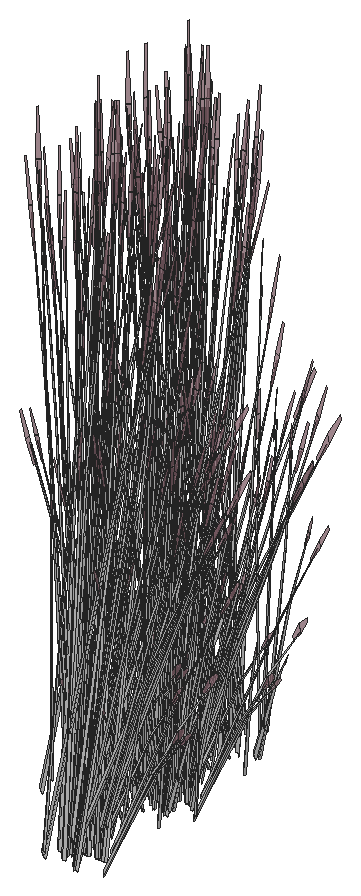
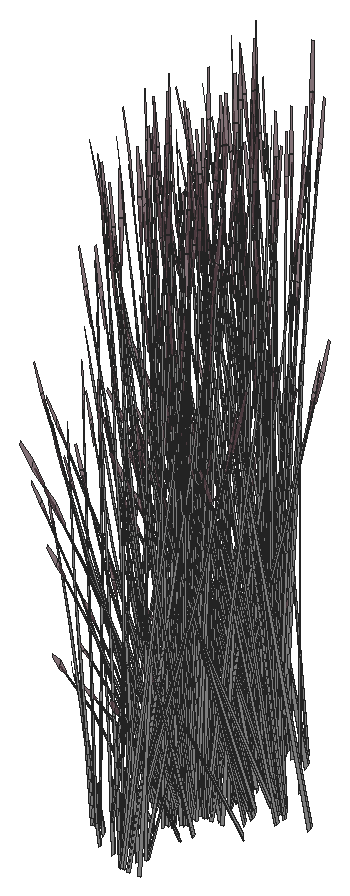
# SketchUp Ruby script. Lengths in inches.
U = 1.inch
M = Sketchup.active_model
def pt(a) = Geom::Point3d.new(a.map { |v| v * U })
def face(e, loops, mat)
  f = e.add_face(loops[0].map { |a| pt(a) })
  loops[1..].each { |l| e.add_face(l.map { |a| pt(a) }).erase! }
  f.material = f.back_material = mat if mat
  f
end
# faces: each face lists its corners as indices into pts; further lists are holes
def faces(e, pts, list, mat = nil) = list.each { |f| face(e, (f[0].is_a?(Array) ? f : [f]).map { |l| l.map { |i| pts[i] } }, mat) }
# xy, xz, yz: faces in a plane at the given z, y or x. An outline is a flat list of corners, or four numbers for a rectangle; further outlines are holes
def ring(l) = l.size == 4 ? [[l[0], l[1]], [l[2], l[1]], [l[2], l[3]], [l[0], l[3]]] : l.each_slice(2).to_a
def flat(e, list, mat, &to3) = list.each { |f| face(e, (f[0].is_a?(Array) ? f : [f]).map { |l| ring(l).map { |u, v| to3.(u, v) } }, mat) }
def xy(e, z, list, mat = nil) = flat(e, list, mat) { |x, y| [x, y, z] }
def xz(e, y, list, mat = nil) = flat(e, list, mat) { |x, z| [x, y, z] }
def yz(e, x, list, mat = nil) = flat(e, list, mat) { |y, z| [x, y, z] }
def lines(e, pts, list) = list.each { |a, b| e.add_line(pt(pts[a]), pt(pts[b])) }
# prism: a flat outline (further loops are holes) pulled along v
def prism(e, loops, v, mat = nil)
  f = face(e, loops, mat); d = Geom::Vector3d.new(v.map { |x| x * U })
  f.pushpull(f.normal.samedirection?(d) ? d.length : -d.length)
end
def box(e, o, s, mat = nil) = prism(e, [[o, [o[0] + s[0], o[1], o[2]], [o[0] + s[0], o[1] + s[1], o[2]], [o[0], o[1] + s[1], o[2]]]], [0, 0, s[2]], mat)
def at(x, y, z, deg = 0) = Geom::Transformation.translation(pt([x, y, z])) * Geom::Transformation.rotation(ORIGIN, Z_AXIS, deg.degrees)
def axes(o, x, y, z) = Geom::Transformation.new([*x, 0, *y, 0, *z, 0, *pt(o).to_a, 1])
def part(name) = M.definitions.add(name)
# library, detail: a bought-in or finely detailed component or shape, given as its bounding box
def library(name, o, s) = part(name).tap { |d| box(d.entities, o, s) }
def detail(e, o, s) = box(e.add_group.entities, o, s)
def put(e, d, t, mat = nil) = e.add_instance(d, t).tap { |i| i.material = mat if mat }
def group(e, t, mat = nil) = e.add_group.tap { |g| g.transformation = t; g.material = mat if mat }.entities
root = M.entities
M.materials.add("LightPink_Translucent").color = [144, 107, 117]
M.materials["LightPink_Translucent"].alpha = 0.75
M.materials.add("[_0053_Ivory_]").color = [200, 200, 200]
c1 = part("blade")
p = [[2.15,0.21,22],[0,0.17,0],[0.09,0.45,0],[2.18,0.31,22],[2.29,0.31,22],[0.38,0.45,0],
  [2.48,0.24,33],[2.49,0.24,33],[2.48,0.22,33]]
faces(c1.entities,p,[[0,1,2,3],[4,5,2,3],[6,3,4,7],[8,0,3,6]])
c2 = part("seeds")
p = [[0.3,-0.1,1.38],[-0.01,-0.03,1.59],[-0.01,-0.03,0.03],[0.14,-0.07,-0.07],[0.29,-0.03,3],[0.15,0.01,3.11]]
faces(c2.entities,p,[[0,1,2,3],[1,0,4,5]],"LightPink_Translucent")
c3 = part("blade with seeds")
put(c3.entities,c1,at(0,0,0))
put(c3.entities,c2,axes([2.4,0.25,30.99],[1.5799,-0.05474,1.17369],[-0.12525,1.92788,0.29478],[-0.07173,-0.02425,1.56792]))
put(root,c3,axes([678.38,324.65,38.66],[0.43478,0.42253,-0.5672],[-0.45929,0.37004,-0.43934],[-0.06615,0.21468,1.08528]),"[_0053_Ivory_]")
put(root,c3,axes([680.62,314.26,35.68],[-0.56663,-0.1556,-0.30978],[0.14267,-0.54795,0.30978],[-0.11423,0.06319,1.38974]),"[_0053_Ivory_]")
put(root,c3,axes([680.62,324.85,35.68],[-0.56663,-0.1556,-0.30978],[0.14267,-0.54795,0.30978],[-0.11423,0.06319,1.38974]),"[_0053_Ivory_]")
put(root,c3,axes([674.08,318.79,36.32],[0.61322,-0.4175,-0.29095],[0.40778,0.58992,-0.50002],[0.1513,0.05991,1.59708]),"[_0053_Ivory_]")
put(root,c3,axes([675.55,322.3,36.32],[-0.38947,-0.01972,1.0506],[0.25721,-0.41888,0.58006],[0.15386,0.14882,0.8241]),"[_0053_Ivory_]")
put(root,c3,axes([679.16,322.7,36.32],[-0.68399,-0.30005,-0.29095],[0.32934,-0.63331,-0.50002],[-0.0215,-0.15549,1.59708]),"[_0053_Ivory_]")
put(root,c3,axes([679.16,332.84,36.32],[-0.68399,-0.30005,-0.29095],[0.32934,-0.63331,-0.50002],[-0.0215,-0.15549,1.59708]),"[_0053_Ivory_]")
put(root,c3,axes([680.94,311.92,36.5],[-0.01659,-0.59209,1.41272],[0.75089,0.15348,0.59816],[-0.1776,0.32398,1.3335]),"[_0053_Ivory_]")
put(root,c3,axes([680.94,322.51,36.5],[-0.01659,-0.59209,1.41272],[0.75089,0.15348,0.59816],[-0.1776,0.32398,1.3335]),"[_0053_Ivory_]")
put(root,c3,axes([674.38,317.28,37.53],[-0.11309,0.21615,1.71376],[-0.47441,-0.44731,0.13857],[0.21402,-0.27879,0.73262]),"[_0053_Ivory_]")
put(root,c3,axes([677.91,314.6875,36.48],[0.55175,-0.11136,0.06507],[0.12684,0.44864,-0.86304],[-0.03498,0.22711,0.7736]),"[_0053_Ivory_]")
put(root,c3,axes([677.91,325.28,36.48],[0.55175,-0.11136,0.06507],[0.12684,0.44864,-0.86304],[-0.03498,0.22711,0.7736]),"[_0053_Ivory_]")
put(root,c3,axes([680.52,312.67,36.32],[0.07077,0.71755,-0.29095],[-0.73712,0.04339,-0.50002],[-0.1298,0.09558,1.59708]),"[_0053_Ivory_]")
put(root,c3,axes([680.52,323.26,36.32],[0.07077,0.71755,-0.29095],[-0.73712,0.04339,-0.50002],[-0.1298,0.09558,1.59708]),"[_0053_Ivory_]")
put(root,c3,axes([678.86,322.06,35.75],[-0.24943,-0.64486,-0.69835],[0.71849,-0.23224,-0.18329],[-0.02757,-0.21836,1.54149]),"[_0053_Ivory_]")
put(root,c3,axes([678.86,332.2,35.75],[-0.24943,-0.64486,-0.69835],[0.71849,-0.23224,-0.18329],[-0.02757,-0.21836,1.54149]),"[_0053_Ivory_]")
put(root,c3,axes([679.98,320.04,38.33],[-0.59704,-0.15764,-0.51099],[0.20464,-0.54049,-0.3958],[-0.05475,-0.21761,0.97773]),"[_0053_Ivory_]")
put(root,c3,axes([679.98,330.18,38.33],[-0.59704,-0.15764,-0.51099],[0.20464,-0.54049,-0.3958],[-0.05475,-0.21761,0.97773]),"[_0053_Ivory_]")
put(root,c3,axes([678.88,313.45,37.53],[-0.01487,-0.24136,1.71376],[0.64429,0.16012,0.13857],[-0.03985,0.34396,0.73262]),"[_0053_Ivory_]")
put(root,c3,axes([672.53,318.41,35.25],[-0.59782,0.25177,1.28929],[-0.19028,-0.72239,0.50096],[0.36709,0.01202,1.46642]),"[_0053_Ivory_]")
put(root,c3,axes([677.68,321.98,35.68],[0.42396,-0.39235,-0.30978],[0.42396,0.39235,0.30978],[0,-0.12637,1.38974]),"[_0053_Ivory_]")
put(root,c3,axes([677.68,332.12,35.68],[0.42396,-0.39235,-0.30978],[0.42396,0.39235,0.30978],[0,-0.12637,1.38974]),"[_0053_Ivory_]")
put(root,c3,axes([679.59,319.45,35.78],[-0.4197,0.36076,-0.03893],[-0.38456,-0.39511,-0.17649],[-0.02707,-0.11196,0.58215]),"[_0053_Ivory_]")
put(root,c3,axes([679.59,329.59,35.78],[-0.4197,0.36076,-0.03893],[-0.38456,-0.39511,-0.17649],[-0.02707,-0.11196,0.58215]),"[_0053_Ivory_]")
put(root,c3,axes([679.42,312.41,36.01],[0.76764,0.13249,0.45755],[-0.15622,0.74829,0.17955],[-0.11218,-0.07226,1.58856]),"[_0053_Ivory_]")
put(root,c3,axes([679.42,323,36.01],[0.76764,0.13249,0.45755],[-0.15622,0.74829,0.17955],[-0.11218,-0.07226,1.58856]),"[_0053_Ivory_]")
put(root,c3,axes([674.73,321.73,38.33],[0.59932,-0.14948,-0.51099],[0.10484,0.56611,-0.3958],[0.16097,0.16223,0.97773]),"[_0053_Ivory_]")
put(root,c3,axes([675.28,317.3,36.03],[0.37973,-0.63014,0],[0.6353,0.35142,-0.51607],[0.14469,0.08004,1.63711]),"[_0053_Ivory_]")
put(root,c3,axes([675.91,317.02,35.15],[-0.0909,-0.04954,1.76342],[-0.2335,-0.55347,-0.26939],[0.15752,-0.1502,0.30037]),"[_0053_Ivory_]")
put(root,c3,axes([679.22,322.87,36.37],[-0.29468,0.56664,0.44739],[-0.61229,-0.27271,-0.21531],[0,-0.13062,1.43643]),"[_0053_Ivory_]")
put(root,c3,axes([680.2,320.14,38.63],[-0.28988,-0.51132,-0.71045],[0.59671,-0.28496,0.08574],[-0.06778,-0.24706,1.00501]),"[_0053_Ivory_]")
put(root,c3,axes([680.2,330.28,38.63],[-0.28988,-0.51132,-0.71045],[0.59671,-0.28496,0.08574],[-0.06778,-0.24706,1.00501]),"[_0053_Ivory_]")
put(root,c3,axes([675.625,317.68,35.67],[0.56842,0.31443,-0.49651],[-0.33976,0.56381,0],[0.12946,0.07161,1.57504]),"[_0053_Ivory_]")
put(root,c3,axes([675.6,322.15,35.15],[0.04425,-0.09079,1.76342],[0.55709,-0.26738,-0.26939],[0.16889,0.13839,0.30037]),"[_0053_Ivory_]")
put(root,c3,axes([675.9,318.35,38.33],[-0.15602,-0.5742,-0.51099],[0.59087,-0.10045,-0.3958],[0.16933,-0.15423,0.97773]),"[_0053_Ivory_]")
put(root,c3,axes([679.01,313.61,36.13],[0.65264,-0.16691,0.17642],[0.16115,0.62115,0.35086],[-0.05821,-0.0905,1.60407]),"[_0053_Ivory_]")
put(root,c3,axes([679.01,324.2,36.13],[0.65264,-0.16691,0.17642],[0.16115,0.62115,0.35086],[-0.05821,-0.0905,1.60407]),"[_0053_Ivory_]")
put(root,c3,axes([676.93,321.3125,37.58],[-0.11624,-0.52862,-0.03492],[0.54943,-0.12153,-0.15832],[0.11473,0.03351,0.52218]),"[_0053_Ivory_]")
put(root,c3,axes([679.85,313.71,35.85],[-0.61229,-0.28233,0],[0.29468,-0.58663,0],[0,0,1.62707]),"[_0053_Ivory_]")
put(root,c3,axes([679.85,324.3,35.85],[-0.61229,-0.28233,0],[0.29468,-0.58663,0],[0,0,1.62707]),"[_0053_Ivory_]")
put(root,c3,axes([681.27,314.41,36.03],[0.37973,0.63014,0],[-0.6353,0.35142,-0.51607],[-0.14469,0.08004,1.63711]),"[_0053_Ivory_]")
put(root,c3,axes([681.27,325,36.03],[0.37973,0.63014,0],[-0.6353,0.35142,-0.51607],[-0.14469,0.08004,1.63711]),"[_0053_Ivory_]")
put(root,c3,axes([674.8,318.88,35.71],[0.63179,0.1031,-0.62353],[-0.13332,0.63596,-0.16365],[0.18854,0.07706,1.37633]),"[_0053_Ivory_]")
put(root,c3,axes([677.49,319.25,35.91],[-0.37654,-0.40212,-0.06488],[0.4124,-0.36845,-0.29416],[0.11685,-0.02594,0.97024]),"[_0053_Ivory_]")
put(root,c3,axes([676.62,317.21,36.42],[-0.2023,0.32011,1.1486],[-0.17388,-0.43009,0.84392],[0.16708,-0.10777,0.25299]),"[_0053_Ivory_]")
put(root,c3,axes([680.95,313.64,36.13],[0.17545,-0.62497,0.17642],[0.64204,0.17686,0.35086],[-0.11091,0.00304,1.60407]),"[_0053_Ivory_]")
put(root,c3,axes([680.95,324.23,36.13],[0.17545,-0.62497,0.17642],[0.64204,0.17686,0.35086],[-0.11091,0.00304,1.60407]),"[_0053_Ivory_]")
put(root,c3,axes([680.66,312.8125,36.27],[0.44871,0.37783,0.1448],[-0.37428,0.42627,-0.41347],[-0.10418,0.05763,1.26744]),"[_0053_Ivory_]")
put(root,c3,axes([680.66,323.4,36.27],[0.44871,0.37783,0.1448],[-0.37428,0.42627,-0.41347],[-0.10418,0.05763,1.26744]),"[_0053_Ivory_]")
put(root,c3,axes([680.5,312.34,35.95],[-0.56493,-0.54126,-0.06131],[0.56528,-0.54159,0],[-0.01973,-0.0189,1.75571]),"[_0053_Ivory_]")
put(root,c3,axes([680.5,322.9375,35.95],[-0.56493,-0.54126,-0.06131],[0.56528,-0.54159,0],[-0.01973,-0.0189,1.75571]),"[_0053_Ivory_]")
put(root,c3,axes([680.65,312.53,36.37],[0.65953,-0.03882,0.44739],[0.05964,0.64439,-0.21531],[-0.11807,0.06531,1.43643]),"[_0053_Ivory_]")
put(root,c3,axes([680.65,323.125,36.37],[0.65953,-0.03882,0.44739],[0.05964,0.64439,-0.21531],[-0.11807,0.06531,1.43643]),"[_0053_Ivory_]")
put(root,c3,axes([680.81,314.02,35.98],[0.76036,0.2044,0.30756],[-0.19023,0.7306,-0.36492],[-0.12585,0.09144,1.64885]),"[_0053_Ivory_]")
put(root,c3,axes([680.81,324.61,35.98],[0.76036,0.2044,0.30756],[-0.19023,0.7306,-0.36492],[-0.12585,0.09144,1.64885]),"[_0053_Ivory_]")
put(root,c3,axes([679.7,319,35.15],[-0.10187,0.02266,1.76342],[-0.56336,-0.25503,-0.26939],[0.00945,-0.21273,0.30037]),"[_0053_Ivory_]")
put(root,c3,axes([679.7,329.14,35.15],[-0.10187,0.02266,1.76342],[-0.56336,-0.25503,-0.26939],[0.00945,-0.21273,0.30037]),"[_0053_Ivory_]")
put(root,c3,axes([681.13,313.98,36.13],[0.56842,-0.31443,0.49651],[0.33976,0.56381,0],[-0.12946,0.07161,1.57504]),"[_0053_Ivory_]")
put(root,c3,axes([681.13,324.57,36.13],[0.56842,-0.31443,0.49651],[0.33976,0.56381,0],[-0.12946,0.07161,1.57504]),"[_0053_Ivory_]")
put(root,c3,axes([674.66,320.24,37.53],[-0.2256,-0.10835,1.71376],[0.46687,-0.45453,0.13857],[0.29098,0.20505,0.73262]),"[_0053_Ivory_]")
put(root,c3,axes([680.25,319.7,38.18],[0.1831,-0.48359,-0.35414],[0.53419,0.14105,0.4572],[-0.04898,-0.1947,0.87481]),"[_0053_Ivory_]")
put(root,c3,axes([680.25,329.84,38.18],[0.1831,-0.48359,-0.35414],[0.53419,0.14105,0.4572],[-0.04898,-0.1947,0.87481]),"[_0053_Ivory_]")
put(root,c3,axes([679.36,322.31,36.01],[0.26406,0.70318,0.45755],[-0.7545,0.24452,0.17955],[0.00922,-0.12921,1.58856]),"[_0053_Ivory_]")
put(root,c3,axes([679.24,322.23,35.86],[0.29468,-0.56664,-0.44739],[0.61229,0.27271,0.21531],[0,-0.13062,1.43643]),"[_0053_Ivory_]")
put(root,c3,axes([679.24,332.37,35.86],[0.29468,-0.56664,-0.44739],[0.61229,0.27271,0.21531],[0,-0.13062,1.43643]),"[_0053_Ivory_]")
put(root,c3,axes([679.99,313.46,35.86],[-0.19817,-0.54216,0],[0.56587,-0.18986,0],[0,0,1.54371]),"[_0053_Ivory_]")
put(root,c3,axes([679.99,324.05,35.86],[-0.19817,-0.54216,0],[0.56587,-0.18986,0],[0,0,1.54371]),"[_0053_Ivory_]")
put(root,c3,axes([679.27,314.6,35.15],[0.09829,-0.03422,1.76342],[0.59126,0.18834,-0.26939],[0.01729,0.21228,0.30037]),"[_0053_Ivory_]")
put(root,c3,axes([679.27,325.2,35.15],[0.09829,-0.03422,1.76342],[0.59126,0.18834,-0.26939],[0.01729,0.21228,0.30037]),"[_0053_Ivory_]")
put(root,c3,axes([676.33,318.41,38.18],[0.52868,-0.08987,-0.35414],[0.1396,0.51376,0.4572],[0.1515,-0.13799,0.87481]),"[_0053_Ivory_]")
put(root,c3,axes([679.4,314.8,38.18],[-0.1831,0.48359,-0.35414],[-0.53419,-0.14105,0.4572],[0.04898,0.1947,0.87481]),"[_0053_Ivory_]")
put(root,c3,axes([675.91,318.58,38.63],[0.31725,-0.49618,-0.71045],[0.55593,0.35263,0.08574],[0.18942,-0.17977,1.00501]),"[_0053_Ivory_]")
put(root,c3,axes([675.91,321.25,38.18],[0.34557,0.39372,-0.35414],[-0.39459,0.37271,0.4572],[0.20048,0.05671,0.87481]),"[_0053_Ivory_]")
put(root,c3,axes([680.79,312.39,35.86],[-0.29468,0.56664,-0.44739],[-0.61229,-0.27271,0.21531],[0,0.13062,1.43643]),"[_0053_Ivory_]")
put(root,c3,axes([680.79,322.98,35.86],[-0.29468,0.56664,-0.44739],[-0.61229,-0.27271,0.21531],[0,0.13062,1.43643]),"[_0053_Ivory_]")
put(root,c3,axes([681.95,312.05,36.13],[-0.47719,-0.45806,0.17642],[0.48088,-0.44429,0.35086],[-0.0527,0.09355,1.60407]),"[_0053_Ivory_]")
put(root,c3,axes([681.95,322.64,36.13],[-0.47719,-0.45806,0.17642],[0.48088,-0.44429,0.35086],[-0.0527,0.09355,1.60407]),"[_0053_Ivory_]")
put(root,c3,axes([680.31,322.375,35.86],[0,-0.72763,0],[0.75945,0,0],[0,0,1.79456]),"[_0053_Ivory_]")
put(root,c3,axes([679.6,322.51,36.09],[0.68433,0.30479,0.24065],[-0.32934,0.63331,0.50002],[0,-0.14599,1.60543]),"[_0053_Ivory_]")
put(root,c3,axes([680.6875,312.07,35.95],[0,0.72727,-0.05637],[-0.75945,0,0],[0,0.02286,1.79368]),"[_0053_Ivory_]")
put(root,c3,axes([680.6875,322.66,35.95],[0,0.72727,-0.05637],[-0.75945,0,0],[0,0.02286,1.79368]),"[_0053_Ivory_]")
put(root,c3,axes([679.38,322.08,36.37],[-0.65953,0.03882,0.44739],[-0.05964,-0.64439,-0.21531],[0.11807,-0.06531,1.43643]),"[_0053_Ivory_]")
put(root,c3,axes([676.17,319.625,38.33],[0.16454,-0.57202,-0.51099],[0.56413,0.19607,-0.3958],[0.22713,-0.05245,0.97773]),"[_0053_Ivory_]")
put(root,c3,axes([677.59,319.99,36.42],[-0.37526,0.10382,1.1486],[0.17664,-0.42906,0.84392],[0.19907,0.02936,0.25299]),"[_0053_Ivory_]")
put(root,c3,axes([679.07,310.38,36.13],[-0.17545,0.62497,0.17642],[-0.64204,-0.17686,0.35086],[0.11091,-0.00304,1.60407]),"[_0053_Ivory_]")
put(root,c3,axes([679.07,320.98,36.13],[-0.17545,0.62497,0.17642],[-0.64204,-0.17686,0.35086],[0.11091,-0.00304,1.60407]),"[_0053_Ivory_]")
put(root,c3,axes([680.32,313.48,35.94],[0.26406,0.72244,-0.06012],[-0.7545,0.25315,0],[0.00922,0.02523,1.72173]),"[_0053_Ivory_]")
put(root,c3,axes([680.32,324.07,35.94],[0.26406,0.72244,-0.06012],[-0.7545,0.25315,0],[0.00922,0.02523,1.72173]),"[_0053_Ivory_]")
put(root,c3,axes([676.37,318.125,36.24],[-0.21697,-0.01863,1.43002],[-0.22228,-0.49966,-0.30754],[0.26655,-0.14135,0.61141]),"[_0053_Ivory_]")
put(root,c3,axes([676.52,319.89,38.18],[0.50475,0.17543,-0.35414],[-0.14722,0.5118,0.4572],[0.20322,-0.04693,0.87481]),"[_0053_Ivory_]")
put(root,c3,axes([678.76,320.2,36.03],[-0.37973,-0.63014,0],[0.6353,-0.35142,-0.51607],[0.14469,-0.08004,1.63711]),"[_0053_Ivory_]")
put(root,c3,axes([678.76,330.34,36.03],[-0.37973,-0.63014,0],[0.6353,-0.35142,-0.51607],[0.14469,-0.08004,1.63711]),"[_0053_Ivory_]")
put(root,c3,axes([679.46,314.36,38.63],[0.28988,0.51132,-0.71045],[-0.59671,0.28496,0.08574],[0.06778,0.24706,1.00501]),"[_0053_Ivory_]")
put(root,c3,axes([682.51,312.53,35.85],[-0.75908,-0.00503,-0.04976],[0,-0.70283,0.49943],[-0.02386,0.16,1.58352]),"[_0053_Ivory_]")
put(root,c3,axes([682.51,323.125,35.85],[-0.75908,-0.00503,-0.04976],[0,-0.70283,0.49943],[-0.02386,0.16,1.58352]),"[_0053_Ivory_]")
put(root,c3,axes([675.54,320.99,38.63],[0.60713,0.01514,-0.71045],[-0.04078,0.63759,0.08574],[0.25721,0.06729,1.00501]),"[_0053_Ivory_]")
put(root,c3,axes([681.01,310.42,36.13],[-0.65264,0.16691,0.17642],[-0.16115,-0.62115,0.35086],[0.05821,0.0905,1.60407]),"[_0053_Ivory_]")
put(root,c3,axes([681.01,321.01,36.13],[-0.65264,0.16691,0.17642],[-0.16115,-0.62115,0.35086],[0.05821,0.0905,1.60407]),"[_0053_Ivory_]")
put(root,c3,axes([676.77,319.79,35.64],[-0.39118,0.07547,1.41583],[-0.06226,-0.6007,0.08104],[0.27398,-0.09092,0.80566]),"[_0053_Ivory_]")
put(root,c3,axes([680.35,318.68,36.42],[0.07791,0.3667,1.1486],[-0.43222,-0.2031,0.84392],[0.04651,-0.18776,0.25299]),"[_0053_Ivory_]")
put(root,c3,axes([680.35,328.82,36.42],[0.07791,0.3667,1.1486],[-0.43222,-0.2031,0.84392],[0.04651,-0.18776,0.25299]),"[_0053_Ivory_]")
put(root,c3,axes([677.2,319.39,35.15],[-0.03174,-0.09547,1.76342],[0.22015,-0.55846,-0.26939],[0.22208,-0.00803,0.30037]),"[_0053_Ivory_]")
put(root,c3,axes([679.95,311.32,36.01],[-0.50358,0.57069,0.45755],[-0.59827,-0.50377,0.17955],[0.1214,-0.05695,1.58856]),"[_0053_Ivory_]")
put(root,c3,axes([679.95,321.92,36.01],[-0.50358,0.57069,0.45755],[-0.59827,-0.50377,0.17955],[0.1214,-0.05695,1.58856]),"[_0053_Ivory_]")
put(root,c3,axes([675.14,319.25,37.53],[-0.25192,0.01424,1.71376],[0.16712,-0.61729,0.13857],[0.35901,0.03818,0.73262]),"[_0053_Ivory_]")
put(root,c3,axes([680.81,312.22,35.87],[0.42396,0.40619,0],[-0.42396,0.40619,0],[0,0,1.69266]),"[_0053_Ivory_]")
put(root,c3,axes([680.81,322.82,35.87],[0.42396,0.40619,0],[-0.42396,0.40619,0],[0,0,1.69266]),"[_0053_Ivory_]")
put(root,c3,axes([680.8,311.75,36.37],[0.29468,-0.56664,0.44739],[0.61229,0.27271,-0.21531],[0,0.13062,1.43643]),"[_0053_Ivory_]")
put(root,c3,axes([680.8,322.34,36.37],[0.29468,-0.56664,0.44739],[0.61229,0.27271,-0.21531],[0,0.13062,1.43643]),"[_0053_Ivory_]")
put(root,c3,axes([680.55,313.72,35.86],[0.61229,0.28233,0],[-0.29468,0.58663,0],[0,0,1.74954]),"[_0053_Ivory_]")
put(root,c3,axes([680.55,324.31,35.86],[0.61229,0.28233,0],[-0.29468,0.58663,0],[0,0,1.74954]),"[_0053_Ivory_]")
put(root,c3,axes([679.67,314.46,38.33],[0.59704,0.15764,-0.51099],[-0.20464,0.54049,-0.3958],[0.05475,0.21761,0.97773]),"[_0053_Ivory_]")
put(root,c3,axes([679.67,325.06,38.33],[0.59704,0.15764,-0.51099],[-0.20464,0.54049,-0.3958],[0.05475,0.21761,0.97773]),"[_0053_Ivory_]")
put(root,c3,axes([680.6,311.61,36.03],[-0.76764,-0.13249,0.49198],[0.15622,-0.74829,0.19306],[0.11218,0.07226,1.70813]),"[_0053_Ivory_]")
put(root,c3,axes([680.6,322.21,36.03],[-0.76764,-0.13249,0.49198],[0.15622,-0.74829,0.19306],[0.11218,0.07226,1.70813]),"[_0053_Ivory_]")
put(root,c3,axes([676.0625,319.83,38.63],[0.53369,-0.27773,-0.71045],[0.29743,0.5717,0.08574],[0.25786,-0.06494,1.00501]),"[_0053_Ivory_]")
put(root,c3,axes([682.35,312.63,35.68],[-0.42396,0.39235,-0.30978],[-0.42396,-0.39235,0.30978],[0,0.12637,1.38974]),"[_0053_Ivory_]")
put(root,c3,axes([682.35,323.23,35.68],[-0.42396,0.39235,-0.30978],[-0.42396,-0.39235,0.30978],[0,0.12637,1.38974]),"[_0053_Ivory_]")
put(root,c3,axes([681.14,312.5625,35.75],[0.2227,0.57576,-0.69212],[-0.64151,0.20736,-0.18165],[0.02462,0.19497,1.52773]),"[_0053_Ivory_]")
put(root,c3,axes([681.14,323.15,35.75],[0.2227,0.57576,-0.69212],[-0.64151,0.20736,-0.18165],[0.02462,0.19497,1.52773]),"[_0053_Ivory_]")
put(root,c3,axes([680.82,311.94,35.86],[0.67951,0,0],[0,0.65103,0],[0,0,1.78407]),"[_0053_Ivory_]")
put(root,c3,axes([680.82,322.54,35.86],[0.67951,0,0],[0,0.65103,0],[0,0,1.78407]),"[_0053_Ivory_]")
put(root,c3,axes([680.17,311.23,36.37],[-0.36485,-0.52782,0.44739],[0.55265,-0.37168,-0.21531],[0.11807,0.06531,1.43643]),"[_0053_Ivory_]")
put(root,c3,axes([680.17,321.82,36.37],[-0.36485,-0.52782,0.44739],[0.55265,-0.37168,-0.21531],[0.11807,0.06531,1.43643]),"[_0053_Ivory_]")
put(root,c3,axes([679.5,321.94,36.32],[-0.07077,-0.71755,-0.29095],[0.73712,-0.04339,-0.50002],[0.1298,-0.09558,1.59708]),"[_0053_Ivory_]")
put(root,c3,axes([679.5,332.08,36.32],[-0.07077,-0.71755,-0.29095],[0.73712,-0.04339,-0.50002],[0.1298,-0.09558,1.59708]),"[_0053_Ivory_]")
put(root,c3,axes([681.06,311.88,36.27],[0.56587,-0.18339,0.1448],[0.19817,0.52368,-0.41347],[0,0.11525,1.26744]),"[_0053_Ivory_]")
put(root,c3,axes([681.06,322.47,36.27],[0.56587,-0.18339,0.1448],[0.19817,0.52368,-0.41347],[0,0.11525,1.26744]),"[_0053_Ivory_]")
put(root,c3,axes([681.27,320.45,38.33],[-0.43478,-0.42253,-0.51099],[0.45929,-0.37004,-0.3958],[0.06615,-0.21468,0.97773]),"[_0053_Ivory_]")
put(root,c3,axes([681.27,330.58,38.33],[-0.43478,-0.42253,-0.51099],[0.45929,-0.37004,-0.3958],[0.06615,-0.21468,0.97773]),"[_0053_Ivory_]")
put(root,c3,axes([676.88,320.68,36.24],[-0.14627,-0.15466,1.43002],[0.19032,-0.51164,-0.30754],[0.29594,0.06931,0.61141]),"[_0053_Ivory_]")
put(root,c3,axes([680.86,311.92,36.32],[0.68399,0.30005,-0.29095],[-0.32934,0.63331,-0.50002],[0.0215,0.15549,1.59708]),"[_0053_Ivory_]")
put(root,c3,axes([680.86,322.51,36.32],[0.68399,0.30005,-0.29095],[-0.32934,0.63331,-0.50002],[0.0215,0.15549,1.59708]),"[_0053_Ivory_]")
put(root,c3,axes([679.41,320.36,35.68],[0.56663,0.1556,-0.30978],[-0.14267,0.54795,0.30978],[0.11423,-0.06319,1.38974]),"[_0053_Ivory_]")
put(root,c3,axes([680.98,319.7,36.24],[-0.17264,0.12729,1.43002],[-0.51703,-0.22279,-0.30754],[0.09584,-0.27707,0.61141]),"[_0053_Ivory_]")
put(root,c3,axes([680.98,329.84,36.24],[-0.17264,0.12729,1.43002],[-0.51703,-0.22279,-0.30754],[0.09584,-0.27707,0.61141]),"[_0053_Ivory_]")
put(root,c3,axes([682.35,312.0625,36.13],[0,-0.62885,0.49651],[0.67951,0,0],[0,0.14322,1.57504]),"[_0053_Ivory_]")
put(root,c3,axes([682.35,322.66,36.13],[0,-0.62885,0.49651],[0.67951,0,0],[0,0.14322,1.57504]),"[_0053_Ivory_]")
put(root,c3,axes([682.64,312.65,35.67],[0,0.62885,-0.49651],[-0.67951,0,0],[0,0.14322,1.57504]),"[_0053_Ivory_]")
put(root,c3,axes([682.64,323.24,35.67],[0,0.62885,-0.49651],[-0.67951,0,0],[0,0.14322,1.57504]),"[_0053_Ivory_]")
put(root,c3,axes([679.27,320.11,35.67],[0.56842,-0.31443,-0.49651],[0.33976,0.56381,0],[0.12946,-0.07161,1.57504]),"[_0053_Ivory_]")
put(root,c3,axes([679.27,330.25,35.67],[0.56842,-0.31443,-0.49651],[0.33976,0.56381,0],[0.12946,-0.07161,1.57504]),"[_0053_Ivory_]")
put(root,c3,axes([680.01,313.35,37.53],[-0.13883,-0.2019,1.71376],[0.64153,-0.16998,0.13857],[0.14499,0.31697,0.73262]),"[_0053_Ivory_]")
put(root,c3,axes([680.01,323.94,37.53],[-0.13883,-0.2019,1.71376],[0.64153,-0.16998,0.13857],[0.14499,0.31697,0.73262]),"[_0053_Ivory_]")
put(root,c3,axes([680.41,311.08,36.27],[0.11717,-0.56122,0.1448],[0.57245,0.09742,-0.41347],[0.10418,0.05763,1.26744]),"[_0053_Ivory_]")
put(root,c3,axes([680.41,321.67,36.27],[0.11717,-0.56122,0.1448],[0.57245,0.09742,-0.41347],[0.10418,0.05763,1.26744]),"[_0053_Ivory_]")
put(root,c3,axes([681.23,320.69,36.13],[-0.56842,-0.31443,0.49651],[0.33976,-0.56381,0],[0.12946,0.07161,1.57504]),"[_0053_Ivory_]")
put(root,c3,axes([681.4,320.64,38.63],[0.0158,-0.58168,-0.71045],[0.66548,0.03907,0.08574],[0.07023,-0.24643,1.00501]),"[_0053_Ivory_]")
put(root,c3,axes([681.4,330.78,38.63],[0.0158,-0.58168,-0.71045],[0.66548,0.03907,0.08574],[0.07023,-0.24643,1.00501]),"[_0053_Ivory_]")
put(root,c3,axes([680.73,313.38,35.84],[0.63764,-0.21337,-0.19198],[0.22406,0.61462,0.00008],[0.07038,-0.02358,1.73897]),"[_0053_Ivory_]")
put(root,c3,axes([680.73,323.98,35.84],[0.63764,-0.21337,-0.19198],[0.22406,0.61462,0.00008],[0.07038,-0.02358,1.73897]),"[_0053_Ivory_]")
put(root,c3,axes([680.74,311.56,35.86],[0.36485,0.52782,-0.44739],[-0.55265,0.37168,0.21531],[0.11807,0.06531,1.43643]),"[_0053_Ivory_]")
put(root,c3,axes([680.74,322.15,35.86],[0.36485,0.52782,-0.44739],[-0.55265,0.37168,0.21531],[0.11807,0.06531,1.43643]),"[_0053_Ivory_]")
put(root,c3,axes([681.68,320.29,38.18],[0.41095,-0.33109,-0.35414],[0.38901,0.37805,0.4572],[0.05919,-0.19208,0.87481]),"[_0053_Ivory_]")
put(root,c3,axes([681.68,330.43,38.18],[0.41095,-0.33109,-0.35414],[0.38901,0.37805,0.4572],[0.05919,-0.19208,0.87481]),"[_0053_Ivory_]")
put(root,c3,axes([681.78,313.95,36.42],[-0.34197,-0.18082,1.1486],[0.44156,-0.18372,0.84392],[0.1191,0.15563,0.25299]),"[_0053_Ivory_]")
put(root,c3,axes([681.78,324.54,36.42],[-0.34197,-0.18082,1.1486],[0.44156,-0.18372,0.84392],[0.1191,0.15563,0.25299]),"[_0053_Ivory_]")
put(root,c3,axes([680.56,313.76,36.24],[0.01072,-0.20846,1.43002],[0.51218,-0.23285,-0.30754],[0.15811,0.2495,0.61141]),"[_0053_Ivory_]")
put(root,c3,axes([680.56,324.35,36.24],[0.01072,-0.20846,1.43002],[0.51218,-0.23285,-0.30754],[0.15811,0.2495,0.61141]),"[_0053_Ivory_]")
put(root,c3,axes([679.95,321.4,35.71],[0.40909,-0.47266,-0.62353],[0.50819,0.4286,-0.16365],[0.16393,-0.11791,1.37633]),"[_0053_Ivory_]")
put(root,c3,axes([679.95,331.54,35.71],[0.40909,-0.47266,-0.62353],[0.50819,0.4286,-0.16365],[0.16393,-0.11791,1.37633]),"[_0053_Ivory_]")
put(root,c3,axes([681.74,310.38,35.68],[0.14267,0.54795,-0.30978],[-0.56663,0.1556,0.30978],[0.11423,0.06319,1.38974]),"[_0053_Ivory_]")
put(root,c3,axes([681.74,320.98,35.68],[0.14267,0.54795,-0.30978],[-0.56663,0.1556,0.30978],[0.11423,0.06319,1.38974]),"[_0053_Ivory_]")
put(root,c3,axes([682.81,312.17,36.03],[0.75945,0,0],[0,0.70283,-0.51607],[0,0.16007,1.63711]),"[_0053_Ivory_]")
put(root,c3,axes([682.81,322.76,36.03],[0.75945,0,0],[0,0.70283,-0.51607],[0,0.16007,1.63711]),"[_0053_Ivory_]")
put(root,c3,axes([680.35,311.26,36.32],[0.61322,-0.4175,-0.29095],[0.40778,0.58992,-0.50002],[0.1513,0.05991,1.59708]),"[_0053_Ivory_]")
put(root,c3,axes([680.35,321.85,36.32],[0.61322,-0.4175,-0.29095],[0.40778,0.58992,-0.50002],[0.1513,0.05991,1.59708]),"[_0053_Ivory_]")
put(root,c3,axes([681.83,314.77,36.32],[-0.38947,-0.01972,1.0506],[0.25721,-0.41888,0.58006],[0.15386,0.14882,0.8241]),"[_0053_Ivory_]")
put(root,c3,axes([681.83,325.37,36.32],[-0.38947,-0.01972,1.0506],[0.25721,-0.41888,0.58006],[0.15386,0.14882,0.8241]),"[_0053_Ivory_]")
put(root,c3,axes([680.65,320.34,37.53],[-0.11309,0.21615,1.71376],[-0.47441,-0.44731,0.13857],[0.21402,-0.27879,0.73262]),"[_0053_Ivory_]")
put(root,c3,axes([680.65,330.48,37.53],[-0.11309,0.21615,1.71376],[-0.47441,-0.44731,0.13857],[0.21402,-0.27879,0.73262]),"[_0053_Ivory_]")
put(root,c3,axes([678.81,310.89,35.25],[-0.59782,0.25177,1.28929],[-0.19028,-0.72239,0.50096],[0.36709,0.01202,1.46642]),"[_0053_Ivory_]")
put(root,c3,axes([678.81,321.48,35.25],[-0.59782,0.25177,1.28929],[-0.19028,-0.72239,0.50096],[0.36709,0.01202,1.46642]),"[_0053_Ivory_]")
put(root,c3,axes([681,314.2,38.33],[0.59932,-0.14948,-0.51099],[0.10484,0.56611,-0.3958],[0.16097,0.16223,0.97773]),"[_0053_Ivory_]")
put(root,c3,axes([681,324.79,38.33],[0.59932,-0.14948,-0.51099],[0.10484,0.56611,-0.3958],[0.16097,0.16223,0.97773]),"[_0053_Ivory_]")
put(root,c3,axes([681.55,320.36,36.03],[0.37973,-0.63014,0],[0.6353,0.35142,-0.51607],[0.14469,0.08004,1.63711]),"[_0053_Ivory_]")
put(root,c3,axes([682.19,320.09,35.15],[-0.0909,-0.04954,1.76342],[-0.2335,-0.55347,-0.26939],[0.15752,-0.1502,0.30037]),"[_0053_Ivory_]")
put(root,c3,axes([682.19,330.23,35.15],[-0.0909,-0.04954,1.76342],[-0.2335,-0.55347,-0.26939],[0.15752,-0.1502,0.30037]),"[_0053_Ivory_]")
put(root,c3,axes([681.9,310.15,35.67],[0.56842,0.31443,-0.49651],[-0.33976,0.56381,0],[0.12946,0.07161,1.57504]),"[_0053_Ivory_]")
put(root,c3,axes([681.9,320.74,35.67],[0.56842,0.31443,-0.49651],[-0.33976,0.56381,0],[0.12946,0.07161,1.57504]),"[_0053_Ivory_]")
put(root,c3,axes([681.87,314.625,35.15],[0.04425,-0.09079,1.76342],[0.55709,-0.26738,-0.26939],[0.16889,0.13839,0.30037]),"[_0053_Ivory_]")
put(root,c3,axes([681.87,325.22,35.15],[0.04425,-0.09079,1.76342],[0.55709,-0.26738,-0.26939],[0.16889,0.13839,0.30037]),"[_0053_Ivory_]")
put(root,c3,axes([682.17,321.42,38.33],[-0.15602,-0.5742,-0.51099],[0.59087,-0.10045,-0.3958],[0.16933,-0.15423,0.97773]),"[_0053_Ivory_]")
put(root,c3,axes([682.17,331.56,38.33],[-0.15602,-0.5742,-0.51099],[0.59087,-0.10045,-0.3958],[0.16933,-0.15423,0.97773]),"[_0053_Ivory_]")
put(root,c3,axes([683.21,313.79,37.58],[-0.11624,-0.52862,-0.03492],[0.54943,-0.12153,-0.15832],[0.11473,0.03351,0.52218]),"[_0053_Ivory_]")
put(root,c3,axes([683.21,324.38,37.58],[-0.11624,-0.52862,-0.03492],[0.54943,-0.12153,-0.15832],[0.11473,0.03351,0.52218]),"[_0053_Ivory_]")
put(root,c3,axes([681.07,311.35,35.71],[0.63179,0.1031,-0.62353],[-0.13332,0.63596,-0.16365],[0.18854,0.07706,1.37633]),"[_0053_Ivory_]")
put(root,c3,axes([681.07,321.95,35.71],[0.63179,0.1031,-0.62353],[-0.13332,0.63596,-0.16365],[0.18854,0.07706,1.37633]),"[_0053_Ivory_]")
put(root,c3,axes([683.76,322.32,35.91],[-0.37654,-0.40212,-0.06488],[0.4124,-0.36845,-0.29416],[0.11685,-0.02594,0.97024]),"[_0053_Ivory_]")
put(root,c3,axes([682.9,320.28,36.42],[-0.2023,0.32011,1.1486],[-0.17388,-0.43009,0.84392],[0.16708,-0.10777,0.25299]),"[_0053_Ivory_]")
put(root,c3,axes([682.9,330.42,36.42],[-0.2023,0.32011,1.1486],[-0.17388,-0.43009,0.84392],[0.16708,-0.10777,0.25299]),"[_0053_Ivory_]")
put(root,c3,axes([680.94,312.72,37.53],[-0.2256,-0.10835,1.71376],[0.46687,-0.45453,0.13857],[0.29098,0.20505,0.73262]),"[_0053_Ivory_]")
put(root,c3,axes([680.94,323.3125,37.53],[-0.2256,-0.10835,1.71376],[0.46687,-0.45453,0.13857],[0.29098,0.20505,0.73262]),"[_0053_Ivory_]")
put(root,c3,axes([682.61,321.48,38.18],[0.52868,-0.08987,-0.35414],[0.1396,0.51376,0.4572],[0.1515,-0.13799,0.87481]),"[_0053_Ivory_]")
put(root,c3,axes([682.61,331.62,38.18],[0.52868,-0.08987,-0.35414],[0.1396,0.51376,0.4572],[0.1515,-0.13799,0.87481]),"[_0053_Ivory_]")
put(root,c3,axes([682.1875,321.65,38.63],[0.31725,-0.49618,-0.71045],[0.55593,0.35263,0.08574],[0.18942,-0.17977,1.00501]),"[_0053_Ivory_]")
put(root,c3,axes([682.1875,331.79,38.63],[0.31725,-0.49618,-0.71045],[0.55593,0.35263,0.08574],[0.18942,-0.17977,1.00501]),"[_0053_Ivory_]")
put(root,c3,axes([682.18,313.73,38.18],[0.34557,0.39372,-0.35414],[-0.39459,0.37271,0.4572],[0.20048,0.05671,0.87481]),"[_0053_Ivory_]")
put(root,c3,axes([682.18,324.32,38.18],[0.34557,0.39372,-0.35414],[-0.39459,0.37271,0.4572],[0.20048,0.05671,0.87481]),"[_0053_Ivory_]")
put(root,c3,axes([682.45,322.69,38.33],[0.16454,-0.57202,-0.51099],[0.56413,0.19607,-0.3958],[0.22713,-0.05245,0.97773]),"[_0053_Ivory_]")
put(root,c3,axes([683.86,312.46,36.42],[-0.37526,0.10382,1.1486],[0.17664,-0.42906,0.84392],[0.19907,0.02936,0.25299]),"[_0053_Ivory_]")
put(root,c3,axes([683.86,323.06,36.42],[-0.37526,0.10382,1.1486],[0.17664,-0.42906,0.84392],[0.19907,0.02936,0.25299]),"[_0053_Ivory_]")
put(root,c3,axes([682.65,321.19,36.24],[-0.21697,-0.01863,1.43002],[-0.22228,-0.49966,-0.30754],[0.26655,-0.14135,0.61141]),"[_0053_Ivory_]")
put(root,c3,axes([682.65,331.33,36.24],[-0.21697,-0.01863,1.43002],[-0.22228,-0.49966,-0.30754],[0.26655,-0.14135,0.61141]),"[_0053_Ivory_]")
put(root,c3,axes([682.79,312.36,38.18],[0.50475,0.17543,-0.35414],[-0.14722,0.5118,0.4572],[0.20322,-0.04693,0.87481]),"[_0053_Ivory_]")
put(root,c3,axes([682.79,322.95,38.18],[0.50475,0.17543,-0.35414],[-0.14722,0.5118,0.4572],[0.20322,-0.04693,0.87481]),"[_0053_Ivory_]")
put(root,c3,axes([681.82,313.46,38.63],[0.60713,0.01514,-0.71045],[-0.04078,0.63759,0.08574],[0.25721,0.06729,1.00501]),"[_0053_Ivory_]")
put(root,c3,axes([681.82,324.06,38.63],[0.60713,0.01514,-0.71045],[-0.04078,0.63759,0.08574],[0.25721,0.06729,1.00501]),"[_0053_Ivory_]")
put(root,c3,axes([683.05,322.85,35.64],[-0.39118,0.07547,1.41583],[-0.06226,-0.6007,0.08104],[0.27398,-0.09092,0.80566]),"[_0053_Ivory_]")
put(root,c3,axes([683.48,311.87,35.15],[-0.03174,-0.09547,1.76342],[0.22015,-0.55846,-0.26939],[0.22208,-0.00803,0.30037]),"[_0053_Ivory_]")
put(root,c3,axes([683.48,322.46,35.15],[-0.03174,-0.09547,1.76342],[0.22015,-0.55846,-0.26939],[0.22208,-0.00803,0.30037]),"[_0053_Ivory_]")
put(root,c3,axes([681.42,311.73,37.53],[-0.25192,0.01424,1.71376],[0.16712,-0.61729,0.13857],[0.35901,0.03818,0.73262]),"[_0053_Ivory_]")
put(root,c3,axes([681.42,322.32,37.53],[-0.25192,0.01424,1.71376],[0.16712,-0.61729,0.13857],[0.35901,0.03818,0.73262]),"[_0053_Ivory_]")
put(root,c3,axes([682.34,312.31,38.63],[0.53369,-0.27773,-0.71045],[0.29743,0.5717,0.08574],[0.25786,-0.06494,1.00501]),"[_0053_Ivory_]")
put(root,c3,axes([682.34,322.9,38.63],[0.53369,-0.27773,-0.71045],[0.29743,0.5717,0.08574],[0.25786,-0.06494,1.00501]),"[_0053_Ivory_]")
put(root,c3,axes([683.16,313.15,36.24],[-0.14627,-0.15466,1.43002],[0.19032,-0.51164,-0.30754],[0.29594,0.06931,0.61141]),"[_0053_Ivory_]")
put(root,c3,axes([683.16,323.75,36.24],[-0.14627,-0.15466,1.43002],[0.19032,-0.51164,-0.30754],[0.29594,0.06931,0.61141]),"[_0053_Ivory_]")
